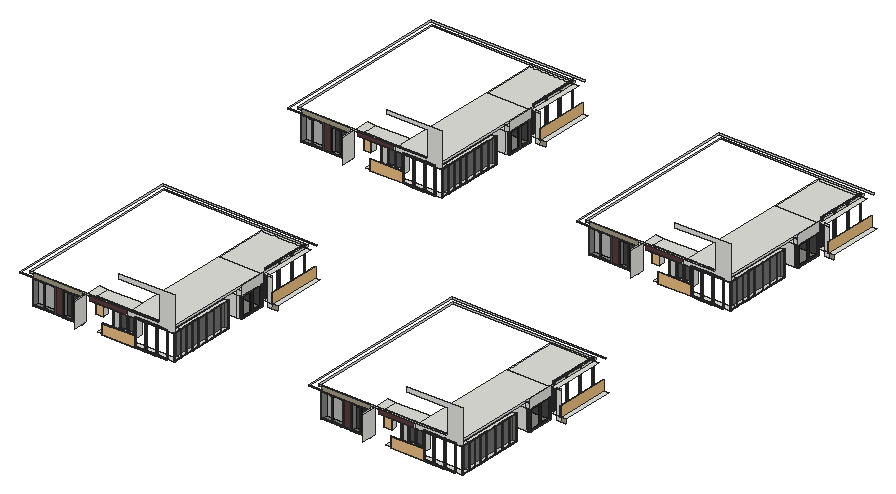
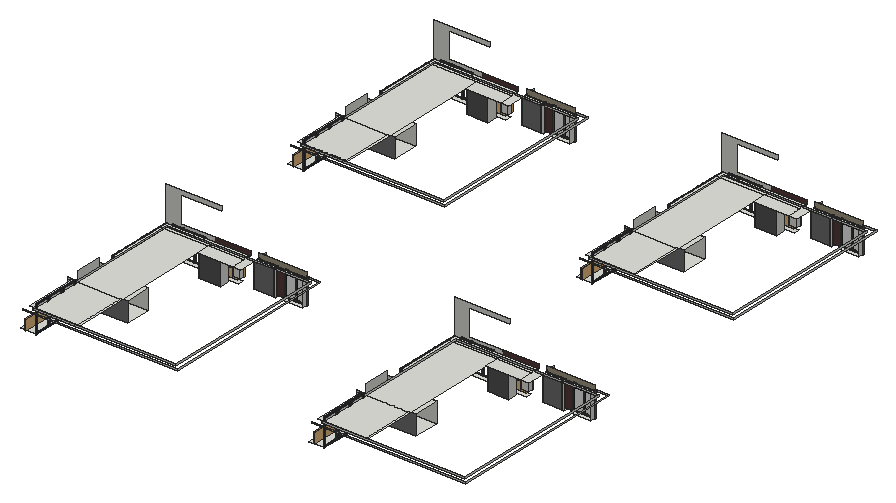
# SketchUp Ruby script. Lengths in inches.
U = 1.inch
M = Sketchup.active_model
def pt(a) = Geom::Point3d.new(a.map { |v| v * U })
def face(e, loops, mat)
  f = e.add_face(loops[0].map { |a| pt(a) })
  loops[1..].each { |l| e.add_face(l.map { |a| pt(a) }).erase! }
  f.material = f.back_material = mat if mat
  f
end
# faces: each face lists its corners as indices into pts; further lists are holes
def faces(e, pts, list, mat = nil) = list.each { |f| face(e, (f[0].is_a?(Array) ? f : [f]).map { |l| l.map { |i| pts[i] } }, mat) }
# xy, xz, yz: faces in a plane at the given z, y or x. An outline is a flat list of corners, or four numbers for a rectangle; further outlines are holes
def ring(l) = l.size == 4 ? [[l[0], l[1]], [l[2], l[1]], [l[2], l[3]], [l[0], l[3]]] : l.each_slice(2).to_a
def flat(e, list, mat, &to3) = list.each { |f| face(e, (f[0].is_a?(Array) ? f : [f]).map { |l| ring(l).map { |u, v| to3.(u, v) } }, mat) }
def xy(e, z, list, mat = nil) = flat(e, list, mat) { |x, y| [x, y, z] }
def xz(e, y, list, mat = nil) = flat(e, list, mat) { |x, z| [x, y, z] }
def yz(e, x, list, mat = nil) = flat(e, list, mat) { |y, z| [x, y, z] }
def lines(e, pts, list) = list.each { |a, b| e.add_line(pt(pts[a]), pt(pts[b])) }
# prism: a flat outline (further loops are holes) pulled along v
def prism(e, loops, v, mat = nil)
  f = face(e, loops, mat); d = Geom::Vector3d.new(v.map { |x| x * U })
  f.pushpull(f.normal.samedirection?(d) ? d.length : -d.length)
end
def box(e, o, s, mat = nil) = prism(e, [[o, [o[0] + s[0], o[1], o[2]], [o[0] + s[0], o[1] + s[1], o[2]], [o[0], o[1] + s[1], o[2]]]], [0, 0, s[2]], mat)
def at(x, y, z, deg = 0) = Geom::Transformation.translation(pt([x, y, z])) * Geom::Transformation.rotation(ORIGIN, Z_AXIS, deg.degrees)
def axes(o, x, y, z) = Geom::Transformation.new([*x, 0, *y, 0, *z, 0, *pt(o).to_a, 1])
def part(name) = M.definitions.add(name)
# library, detail: a bought-in or finely detailed component or shape, given as its bounding box
def library(name, o, s) = part(name).tap { |d| box(d.entities, o, s) }
def detail(e, o, s) = box(e.add_group.entities, o, s)
def put(e, d, t, mat = nil) = e.add_instance(d, t).tap { |i| i.material = mat if mat }
def group(e, t, mat = nil) = e.add_group.tap { |g| g.transformation = t; g.material = mat if mat }.entities
root = M.entities
M.materials.add("Glass_Tinted_Gray").color = [0, 0, 0]
M.materials["Glass_Tinted_Gray"].alpha = 0.125
M.materials.add("Glazing").color = [128, 128, 128]
M.materials["Glazing"].alpha = 0.05
M.materials.add("Powdercoating").color = [41, 44, 40]
M.materials.add("Wine2").color = [0, 0, 0]
M.materials["Wine2"].alpha = 0
M.materials.add("[0130_Gainsboro]").color = [39, 45, 50]
M.materials.add("[0135_DarkGray]").color = [81, 81, 81]
M.materials.add("[Color M05]").color = [114, 114, 114]
M.materials.add("[Color M06]").color = [86, 86, 86]
M.materials.add("[Concrete Tile]").color = [165, 155, 133]
M.materials.add("[Granite Brown]").color = [89, 59, 61]
M.materials.add("[Mirror 02]").color = [229, 229, 229]
M.materials.add("[Terrazzo Light Blue]").color = [196, 214, 227]
c1 = part("Framed glazing panel")
xy(c1.entities,0,[[0,-0.98,43.07,0],[0,0,43.07,1.4]],"[0130_Gainsboro]")
xy(c1.entities,0.3,[[0.3,-1.43,42.77,-0.98]],"[0130_Gainsboro]")
xy(c1.entities,2.95,[[2.95,-1.43,40.12,-0.63],[2.95,-0.63,40.12,0],[2.95,0,40.12,0.64],[2.95,0.64,40.12,1.4]],"[0130_Gainsboro]")
xy(c1.entities,3.54,[[3.54,-0.63,39.53,0],[3.54,0,39.53,0.64]],"[0130_Gainsboro]")
xy(c1.entities,111.8125,[[3.54,-0.63,39.53,0],[3.54,0,39.53,0.64]],"[0130_Gainsboro]")
xy(c1.entities,112.4,[[2.95,-1.43,40.12,-0.63],[2.95,-0.63,40.12,0],[2.95,0,40.12,0.64],[2.95,0.64,40.12,1.4]],"[0130_Gainsboro]")
xy(c1.entities,115.05,[[0.3,-1.43,42.77,-0.98]],"[0130_Gainsboro]")
xy(c1.entities,115.35,[[0,-0.98,43.07,0],[0,0,43.07,1.4]],"[0130_Gainsboro]")
xz(c1.entities,-1.43,[[[0.3,0.3,42.77,115.05],[2.95,2.95,40.12,112.4]]],"[0130_Gainsboro]")
xz(c1.entities,-0.98,[[[0,0,43.07,115.35],[0.3,0.3,42.77,115.05]]],"[0130_Gainsboro]")
xz(c1.entities,-0.63,[[[2.95,2.95,40.12,112.4],[3.54,3.54,39.53,111.8125]]],"[0130_Gainsboro]")
xz(c1.entities,0,[[3.54,3.54,39.53,111.8125]],"Wine2")
xz(c1.entities,0,[[[0,0,43.07,115.35],[2.95,2.95,40.12,112.4]],[[2.95,2.95,40.12,112.4],[3.54,3.54,39.53,111.8125]]],"[0130_Gainsboro]")
xz(c1.entities,0.64,[[[2.95,2.95,40.12,112.4],[3.54,3.54,39.53,111.8125]]],"[0130_Gainsboro]")
xz(c1.entities,1.4,[[[0,0,43.07,115.35],[2.95,2.95,40.12,112.4]]],"[0130_Gainsboro]")
yz(c1.entities,0,[[-0.98,0,0,115.35],[0,0,1.4,115.35]],"[0130_Gainsboro]")
yz(c1.entities,0.3,[[-1.43,0.3,-0.98,115.05]],"[0130_Gainsboro]")
yz(c1.entities,2.95,[[-1.43,2.95,-0.63,112.4],[-0.63,2.95,0,112.4],[0,2.95,0.64,112.4],[0.64,2.95,1.4,112.4]],"[0130_Gainsboro]")
yz(c1.entities,3.54,[[-0.63,3.54,0,111.8125],[0,3.54,0.64,111.8125]],"[0130_Gainsboro]")
yz(c1.entities,39.53,[[-0.63,3.54,0,111.8125],[0,3.54,0.64,111.8125]],"[0130_Gainsboro]")
yz(c1.entities,40.12,[[-1.43,2.95,-0.63,112.4],[-0.63,2.95,0,112.4],[0,2.95,0.64,112.4],[0.64,2.95,1.4,112.4]],"[0130_Gainsboro]")
yz(c1.entities,42.77,[[-1.43,0.3,-0.98,115.05]],"[0130_Gainsboro]")
yz(c1.entities,43.07,[[-0.98,0,0,115.35],[0,0,1.4,115.35]],"[0130_Gainsboro]")
c2 = part("Glazed panel assembly")
put(c2.entities,c1,axes([90.57,1.43,0],[1.05148,0,0],[0,1,0],[0,0,1]))
put(c2.entities,c1,axes([0,1.43,0],[1.05148,0,0],[0,1,0],[0,0,1]))
put(c2.entities,c1,axes([45.29,1.43,0],[1.05148,0,0],[0,1,0],[0,0,1]))
c3 = library("Glass Railing",[0,0,0],[139.5,4.76,42])
c4 = part("Group\#15")
xy(c4.entities,0,[[0,-55.94,0.71,45.94]])
xy(c4.entities,0.2,[[0,-55.94,0.47,45.94],[0.47,45.94,0.71,46.42]])
xy(c4.entities,2.36,[[0.47,-55.94,0.71,46.42]])
xz(c4.entities,-55.94,[[0,0,0.71,0,0.71,2.36,0.47,2.36,0.47,0.2,0,0.2]])
xz(c4.entities,45.94,[[0,0,0.71,0.2]])
xz(c4.entities,46.42,[[0.47,0.2,0.71,2.36]])
yz(c4.entities,0,[[-55.94,0,45.94,0.2]])
yz(c4.entities,0.47,[[-55.94,0.2,46.42,2.36]])
yz(c4.entities,0.71,[[-55.94,0,45.94,0,45.94,0.2,46.42,0.2,46.42,2.36,-55.94,2.36]])
c5 = part("Group\#7")
xy(c5.entities,0,[[0,-59.09,0.71,45.94]])
xy(c5.entities,0.2,[[0,-59.09,0.47,45.94],[0.47,45.94,0.71,46.42]])
xy(c5.entities,2.36,[[0.47,-59.09,0.71,46.42]])
xz(c5.entities,-59.09,[[0,0,0.71,0,0.71,2.36,0.47,2.36,0.47,0.2,0,0.2]])
xz(c5.entities,45.94,[[0,0,0.71,0.2]])
xz(c5.entities,46.42,[[0.47,0.2,0.71,2.36]])
yz(c5.entities,0,[[-59.09,0,45.94,0.2]])
yz(c5.entities,0.47,[[-59.09,0.2,46.42,2.36]])
yz(c5.entities,0.71,[[-59.09,0,45.94,0,45.94,0.2,46.42,0.2,46.42,2.36,-59.09,2.36]])
c6 = part("Group\#16")
prism(c6.entities,[[[0.47,-56.18,0.2],[0,-56.18,0.2],[0,-56.18,0],[0.71,-56.18,0],[0.71,-56.18,2.36],[0.47,-56.18,2.36]]],[0,28.68,0])
c7 = part("Group\#10")
box(c7.entities,[-0.73,0,0],[27.99,0.55,102.05])
c8 = part("Group\#18")
xy(c8.entities,0,[[0.47,-56.18,0.47,-55.47,0,-55.47,0,-28.21,1.18,-28.21,1.18,-56.18]])
xy(c8.entities,0.2,[[0.71,-56.18,1.18,-28.21],[0,-55.47,0.47,-28.21],[0.47,-28.21,0.71,-27.74]])
xy(c8.entities,2.36,[[0.47,-56.18,0.71,-27.74]])
xz(c8.entities,-56.18,[[0.47,0,1.18,0,1.18,0.2,0.71,0.2,0.71,2.36,0.47,2.36]])
xz(c8.entities,-55.47,[[0,0,0.47,0.2]])
xz(c8.entities,-28.21,[[0,0,1.18,0.2]])
xz(c8.entities,-27.74,[[0.47,0.2,0.71,2.36]])
yz(c8.entities,0,[[-55.47,0,-28.21,0.2]])
yz(c8.entities,0.47,[[-56.18,0,-55.47,0.2],[-56.18,0.2,-27.74,2.36]])
yz(c8.entities,0.71,[[-56.18,0.2,-27.74,2.36]])
yz(c8.entities,1.18,[[-56.18,0,-28.21,0.2]])
c9 = part("Group\#34")
xy(c9.entities,0,[[-20.45,0,7.76,1.22]])
xy(c9.entities,0.06,[[-20.39,0.06,7.7,1.22]])
xy(c9.entities,0.47,[[-19.98,0,7.28,0.06]])
xy(c9.entities,101.89,[[-19.98,0,7.28,0.06]])
xy(c9.entities,102.3,[[-20.39,0.06,7.7,1.22]])
xy(c9.entities,102.36,[[-20.45,0,7.76,1.22]])
xz(c9.entities,0,[[[-20.45,0,7.76,102.36],[-19.98,0.47,7.28,101.89]]])
xz(c9.entities,0.06,[[[-20.39,0.06,7.7,102.3],[-19.98,0.47,7.28,101.89]]])
xz(c9.entities,1.22,[[[-20.45,0,7.76,102.36],[-20.39,0.06,7.7,102.3]]])
yz(c9.entities,-20.45,[[0,0,1.22,102.36]])
yz(c9.entities,-20.39,[[0.06,0.06,1.22,102.3]])
yz(c9.entities,-19.98,[[0,0.47,0.06,101.89]])
yz(c9.entities,7.28,[[0,0.47,0.06,101.89]])
yz(c9.entities,7.7,[[0.06,0.06,1.22,102.3]])
yz(c9.entities,7.76,[[0,0,1.22,102.36]])
c10 = part("Group\#6")
put(c10.entities,c4,axes([27.97,0,7.875],[1,0,0],[0,0,-1],[0,1,0]),"Powdercoating")
put(c10.entities,c5,axes([0.71,0,6.8],[-1,0,0],[0,0,-0.97687],[0,1,0]),"Powdercoating")
put(c10.entities,c6,axes([-27.5,0,-38.07],[0,0,-1],[-1,0,0],[0,1,0]),"Powdercoating")
put(c10.entities,c7,at(1.12,0.35,-38.39),"Glazing")
put(c10.entities,c8,axes([-27.5,0,63.35],[0,0,1],[-1,0,0],[0,1,0]),"Powdercoating")
put(c10.entities,c9,at(20.6875,1.0625,-38.54),"Powdercoating")
c11 = part("Sliding door assembly")
put(c11.entities,c10,at(-1.18,4.5,38.86))
g1 = group(c11.entities,at(84.74,4.5,38.86))
put(g1,c4,axes([-27.97,0,7.875],[-1,0,0],[0,0,-1],[0,1,0]),"Powdercoating")
put(g1,c5,axes([-0.71,0,6.8],[1,0,0],[0,0,-0.97687],[0,1,0]),"Powdercoating")
put(g1,c6,axes([27.5,0,-38.07],[0,0,-1],[1,0,0],[0,1,0]),"Powdercoating")
put(g1,c7,axes([-1.12,0.35,-38.39],[-1,0,0],[0,1,0],[0,0,1]),"Glazing")
put(g1,c8,axes([27.5,0,63.35],[0,0,1],[1,0,0],[0,1,0]),"Powdercoating")
put(g1,c9,axes([-20.6875,1.0625,-38.54],[-1,0,0],[0,1,0],[0,0,1]),"Powdercoating")
g2 = group(c11.entities,at(56.0625,4.5,38.86))
put(g2,c4,axes([-27.97,0,7.875],[-1,0,0],[0,0,-1],[0,1,0]),"Powdercoating")
put(g2,c6,axes([27.5,0,-38.07],[0,0,-1],[1,0,0],[0,1,0]),"Powdercoating")
put(g2,c7,axes([-1.12,0.35,-38.39],[-1,0,0],[0,1,0],[0,0,1]),"Glazing")
put(g2,c8,axes([27.5,0,63.35],[0,0,1],[1,0,0],[0,1,0]),"Powdercoating")
put(g2,c9,axes([-20.6875,1.0625,-38.54],[-1,0,0],[0,1,0],[0,0,1]),"Powdercoating")
g3 = group(g2,at(-0.71,0,6.8),"Powdercoating")
xy(g3,-45.34,[[0.47,0.2,0.71,2.36]])
xy(g3,-44.88,[[0,0,0.71,0.2]])
xy(g3,57.73,[[0,0,0.71,0,0.71,2.36,0.47,2.36,0.47,0.2,0,0.2]])
xz(g3,0,[[0,-44.88,0.71,57.73]])
xz(g3,0.2,[[0.47,-45.34,0.71,-44.88],[0,-44.88,0.47,57.73]])
xz(g3,2.36,[[0.47,-45.34,0.71,57.73]])
yz(g3,0,[[0,-44.88,0.2,57.73]])
yz(g3,0.47,[[0.2,-45.34,2.36,57.73]])
yz(g3,0.71,[[0.2,-45.34,2.36,-45.34,2.36,57.73,0,57.73,0,-44.88,0.2,-44.88]])
put(c11.entities,c10,axes([-33.94,4.5,38.86],[1.14218,0,0],[0,1,0],[0,0,1]))
c12 = part("sliding door")
put(c12.entities,c11,at(0,-4.5,-0.08))
c13 = part("PENTEK_RP Fineline 50S_Sliding_DoorCase_E1")
box(c13.entities,[0,0,0],[1.51,3.66,99.27],"[0135_DarkGray]")
c14 = part("PENTEK_RP Fineline 50S_SlidingDooe_Case_E2")
box(c14.entities,[0,0,0],[96.25,3.66,1.51],"[0135_DarkGray]")
c15 = part("pentek_RP Fineline 50S_SlidingDoor_Case")
put(c15.entities,c13,at(97.76,0,0))
put(c15.entities,c14,at(1.51,0,0))
put(c15.entities,c13,at(0,0,0))
put(c15.entities,c14,at(1.51,0,97.76))
c16 = part("PENTEK_RP Fineline 50S_SlidingDoor_GlazingBead_2")
box(c16.entities,[0,0,0],[0.56,0.59,94.39],"[0135_DarkGray]")
c17 = part("PENTEK_RP Fineline 50S_SlidingDoor_Glass")
box(c17.entities,[0,0,0],[46.58,0.16,94.39],"Glass_Tinted_Gray")
c18 = part("PENTEK_RP Fineline 50S_SlidingDoor_GlazingBead")
box(c18.entities,[0,0,0],[45.47,0.59,0.56],"[0135_DarkGray]")
c19 = part("PENTEK_RP Fineline 50S_SlidingDoor_Leaf_E1")
xy(c19.entities,0,[[0,0,0.93,1.97],[0.93,1.57,1.49,1.97]],"[0135_DarkGray]")
xy(c19.entities,96.25,[[0,0,0.93,0,0.93,1.57,1.49,1.57,1.49,1.97,0,1.97]],"[0135_DarkGray]")
xz(c19.entities,0,[[0,0,0.93,96.25]],"[0135_DarkGray]")
xz(c19.entities,1.57,[[0.93,0,1.49,95.32],[0.93,95.32,1.49,96.25]],"[0135_DarkGray]")
xz(c19.entities,1.97,[[0,0,1.49,96.25]],"[0135_DarkGray]")
yz(c19.entities,0,[[0,0,1.97,96.25]],"[0135_DarkGray]")
yz(c19.entities,0.93,[[0,0,1.57,0.93],[0,0.93,1.57,95.32],[0,95.32,1.57,96.25]],"[0135_DarkGray]")
yz(c19.entities,1.49,[[1.57,0,1.97,95.32],[1.57,95.32,1.97,96.25]],"[0135_DarkGray]")
c20 = part("PENTEK_RP Fineline 50S_SlidingDoor_Leaf_E2")
xy(c20.entities,0,[[0,0,0,1.57,0.56,1.57,0.56,1.97,46.02,1.97,46.02,1.57,46.58,1.57,46.58,0]],"[0135_DarkGray]")
xy(c20.entities,0.93,[[0,0,46.58,1.57]],"[0135_DarkGray]")
xy(c20.entities,1.49,[[0.56,1.57,46.02,1.97]],"[0135_DarkGray]")
xz(c20.entities,0,[[0,0,46.58,0.93]],"[0135_DarkGray]")
xz(c20.entities,1.57,[[0,0,0.56,0.93],[46.02,0,46.58,0.93],[0.56,0.93,46.02,1.49]],"[0135_DarkGray]")
xz(c20.entities,1.97,[[0.56,0,46.02,1.49]],"[0135_DarkGray]")
yz(c20.entities,0,[[0,0,1.57,0.93]],"[0135_DarkGray]")
yz(c20.entities,0.56,[[1.57,0,1.97,0.93],[1.57,0.93,1.97,1.49]],"[0135_DarkGray]")
yz(c20.entities,46.02,[[1.57,0,1.97,0.93],[1.57,0.93,1.97,1.49]],"[0135_DarkGray]")
yz(c20.entities,46.58,[[0,0,1.57,0.93]],"[0135_DarkGray]")
c21 = part("PENTEK_RP Fineline S_SlidingDoor_Leaf1")
put(c21.entities,c16,at(0.93,0,0.93))
put(c21.entities,c16,at(46.96,0,0.93))
put(c21.entities,c17,at(1.49,1.42,0.93))
put(c21.entities,c18,at(1.49,0,0.93))
put(c21.entities,c17,at(1.49,0.59,0.93),"[Terrazzo Light Blue]")
put(c21.entities,c19,at(0,0,0))
put(c21.entities,c19,axes([48.44,0,0],[-1,0,0],[0,1,0],[0,0,1]))
put(c21.entities,c20,axes([0.93,0,96.25],[1,0,0],[0,1,0],[0,0,-1]))
put(c21.entities,c20,at(0.93,0,0))
put(c21.entities,c18,at(1.49,0,94.77))
c22 = part("PENTEK_RP Fineline 50S_SlidingDoor_Leaf2")
put(c22.entities,c17,at(1.49,1.42,0.93))
put(c22.entities,c18,at(1.49,0,94.77))
put(c22.entities,c16,at(46.96,0,0.93))
put(c22.entities,c17,at(1.49,0.59,0.93),"[Mirror 02]")
put(c22.entities,c16,at(0.93,0,0.93))
put(c22.entities,c19,at(0,0,0))
put(c22.entities,c19,axes([48.44,0,0],[-1,0,0],[0,1,0],[0,0,1]))
put(c22.entities,c18,at(1.49,0,0.93))
put(c22.entities,c20,axes([0.93,0,96.25],[1,0,0],[0,1,0],[0,0,-1]))
put(c22.entities,c20,at(0.93,0,0))
c23 = part("PENTEK - Slimmest Steel Sliding Door / Window\#1")
put(c23.entities,c15,at(0,-1.88,-0.09))
put(c23.entities,c21,at(1.51,-2.27,1.42))
put(c23.entities,c22,at(49.32,-0.3,1.42))
c24 = library("Klein+raam",[128.36,12.7,0],[19.68,5.51,55.12])
xy(root,1276.95,[[646.53,1835.1875,662.84,1873.375],[662.84,1835.1875,664.52,1873.375],[664.52,1835.1875,715.63,1873.375],[1864.72,1835.1875,1881.02,1873.375],[1881.02,1835.1875,1882.71,1873.375],
  [1882.71,1835.1875,1933.82,1873.375],[646.53,3249.875,662.84,3288.0625],[662.84,3249.875,664.52,3288.0625],[664.52,3249.875,715.63,3288.0625],[1864.72,3249.875,1881.02,3288.0625],
  [1881.02,3249.875,1882.71,3288.0625],[1882.71,3249.875,1933.82,3288.0625]])
xy(root,1277.26,[[625.7,1835.1875,646.53,1873.375],[1843.88,1835.1875,1864.72,1873.375],[625.7,3249.875,646.53,3288.0625],[1843.88,3249.875,1864.72,3288.0625]])
xy(root,1278.6875,[[589.79,1799.9375,913.875,1799.9375,913.875,1835.1875,890.875,1835.1875,890.875,1822.9375,589.79,1822.9375],[1807.98,1799.9375,2132.0625,1799.9375,2132.0625,1835.1875,2109.0625,1835.1875,2109.0625,1822.9375,1807.98,1822.9375],[894.3125,1835.1875,913.875,2085.72],[2112.5,1835.1875,2132.0625,2085.72],[589.79,3214.625,913.875,3214.625,913.875,3249.875,890.875,3249.875,890.875,3237.625,589.79,3237.625],
  [1807.98,3214.625,2132.0625,3214.625,2132.0625,3249.875,2109.0625,3249.875,2109.0625,3237.625,1807.98,3237.625],[894.3125,3249.875,913.875,3500.41],[2112.5,3249.875,2132.0625,3500.41]])
xy(root,1281.4375,[[319.53,1799.9375,523.04,1799.9375,523.04,1822.9375,442.15,1822.9375,442.15,1806.5625,404.95,1806.5625,404.95,1822.9375,319.53,1822.9375],[1537.72,1799.9375,1741.23,1799.9375,1741.23,1822.9375,1660.33,1822.9375,1660.33,1806.5625,1623.14,1806.5625,1623.14,1822.9375,1537.72,1822.9375],[431.33,1806.5625,442.15,1822.9375],[1649.52,1806.5625,1660.33,1822.9375],[319.53,3214.625,523.04,3214.625,523.04,3237.625,442.15,3237.625,442.15,3221.25,404.95,3221.25,404.95,3237.625,319.53,3237.625],
  [1537.72,3214.625,1741.23,3214.625,1741.23,3237.625,1660.33,3237.625,1660.33,3221.25,1623.14,3221.25,1623.14,3237.625,1537.72,3237.625],[431.33,3221.25,442.15,3237.625],[1649.52,3221.25,1660.33,3237.625]])
xy(root,1283.36,[[704.25,2156.01,913.875,2266.33],[1922.4375,2156.01,2132.0625,2266.33],[704.25,3570.7,913.875,3681.01],[1922.4375,3570.7,2132.0625,3681.01]])
xy(root,1286.8125,[[890.875,2295.875,954.6875,2518.89],[2109.0625,2295.875,2172.875,2518.89],[890.875,3710.5625,954.6875,3933.57],[2109.0625,3710.5625,2172.875,3933.57]])
xy(root,1321.04,[[557.4,1835.1875,588.66,1854.3125],[1775.59,1835.1875,1806.84,1854.3125],[557.4,3249.875,588.66,3269],[1775.59,3249.875,1806.84,3269]])
xy(root,1369.04,[[704.25,2156.01,913.875,2266.33],[1922.4375,2156.01,2132.0625,2266.33],[704.25,3570.7,913.875,3681.01],[1922.4375,3570.7,2132.0625,3681.01]])
xy(root,1373.32,[[557.4,1835.1875,588.66,1854.3125],[1775.59,1835.1875,1806.84,1854.3125],[557.4,3249.875,588.66,3269],[1775.59,3249.875,1806.84,3269]])
xy(root,1375.08,[[625.7,1835.1875,715.63,1873.375],[1843.88,1835.1875,1933.82,1873.375],[625.7,3249.875,715.63,3288.0625],[1843.88,3249.875,1933.82,3288.0625]])
xy(root,1386,[[319.53,1799.9375,319.53,1822.9375,405.55,1822.9375,405.55,1806.5625,442.15,1806.5625,442.15,1822.9375,523.04,1822.9375,523.04,1799.9375],[557.88,1799.9375,557.88,1822.9375,890.875,1822.9375,890.875,1835.1875,913.875,1835.1875,913.875,1799.9375],[1537.72,1799.9375,1537.72,1822.9375,1623.74,1822.9375,1623.74,1806.5625,1660.33,1806.5625,1660.33,1822.9375,1741.23,1822.9375,1741.23,1799.9375],[1776.07,1799.9375,1776.07,1822.9375,2109.0625,1822.9375,2109.0625,1835.1875,2132.0625,1835.1875,2132.0625,1799.9375],[431.33,1806.5625,442.15,1822.9375],
  [1649.52,1806.5625,1660.33,1822.9375],[523.04,1822.9375,557.88,1822.9375,557.88,1835.1875,557.4,1835.1875,557.4,1893.6875,523.04,1893.6875],[557.88,1822.9375,704.25,1835.1875],[704.25,1822.9375,890.875,1835.1875],[1741.23,1822.9375,1776.07,1822.9375,1776.07,1835.1875,1775.59,1835.1875,1775.59,1893.6875,1741.23,1893.6875],
  [1776.07,1822.9375,1922.4375,1835.1875],[1922.4375,1822.9375,2109.0625,1835.1875],[557.4,1835.1875,704.25,1893.6875],[704.25,1835.1875,890.875,2295.875],[894.3125,1835.1875,913.875,2085.72],
  [1775.59,1835.1875,1922.4375,1893.6875],[1922.4375,1835.1875,2109.0625,2295.875],[2112.5,1835.1875,2132.0625,2085.72],[704.25,2295.875,710.125,2518.89],[710.125,2295.875,890.875,2518.89],
  [890.875,2295.875,913.875,2518.89],[1922.4375,2295.875,1928.3125,2518.89],[1928.3125,2295.875,2109.0625,2518.89],[2109.0625,2295.875,2132.0625,2518.89],[704.25,2518.89,890.875,2531.375],
  [1922.4375,2518.89,2109.0625,2531.375],[319.53,3214.625,319.53,3237.625,405.55,3237.625,405.55,3221.25,442.15,3221.25,442.15,3237.625,523.04,3237.625,523.04,3214.625],[557.88,3214.625,557.88,3237.625,890.875,3237.625,890.875,3249.875,913.875,3249.875,913.875,3214.625],[1537.72,3214.625,1537.72,3237.625,1623.74,3237.625,1623.74,3221.25,1660.33,3221.25,1660.33,3237.625,1741.23,3237.625,1741.23,3214.625],[1776.07,3214.625,1776.07,3237.625,2109.0625,3237.625,2109.0625,3249.875,2132.0625,3249.875,2132.0625,3214.625],
  [431.33,3221.25,442.15,3237.625],[1649.52,3221.25,1660.33,3237.625],[523.04,3237.625,557.88,3237.625,557.88,3249.875,557.4,3249.875,557.4,3308.375,523.04,3308.375],[557.88,3237.625,704.25,3249.875],[704.25,3237.625,890.875,3249.875],
  [1741.23,3237.625,1776.07,3237.625,1776.07,3249.875,1775.59,3249.875,1775.59,3308.375,1741.23,3308.375],[1776.07,3237.625,1922.4375,3249.875],[1922.4375,3237.625,2109.0625,3249.875],[557.4,3249.875,704.25,3308.375],[704.25,3249.875,890.875,3710.5625],
  [894.3125,3249.875,913.875,3500.41],[1775.59,3249.875,1922.4375,3308.375],[1922.4375,3249.875,2109.0625,3710.5625],[2112.5,3249.875,2132.0625,3500.41],[704.25,3710.5625,710.125,3933.57],
  [710.125,3710.5625,890.875,3933.57],[890.875,3710.5625,913.875,3933.57],[1922.4375,3710.5625,1928.3125,3933.57],[1928.3125,3710.5625,2109.0625,3933.57],[2109.0625,3710.5625,2132.0625,3933.57],
  [704.25,3933.57,890.875,3946.0625],[1922.4375,3933.57,2109.0625,3946.0625]])
xz(root,1799.9375,[[262.875,1386,319.53,1392],[708.87,1386,913.875,1386,913.875,1530.6875,679.51,1530.6875,679.51,1512,851.78,1512,851.78,1404.6875,708.87,1404.6875],[1481.0625,1386,1537.72,1392],[1927.06,1386,2132.0625,1386,2132.0625,1530.6875,1897.7,1530.6875,1897.7,1512,2069.97,1512,2069.97,1404.6875,1927.06,1404.6875]])
xz(root,1799.9375,[[319.53,1386,523.04,1407.4375],[1537.72,1386,1741.23,1407.4375]],"[Concrete Tile]")
xz(root,1799.9375,[[557.88,1386,708.87,1404.6875],[1776.07,1386,1927.06,1404.6875]],"[Granite Brown]")
xz(root,1806.5625,[[405.03,1281.4375,442.15,1281.4375,442.15,1386,405.55,1386],[1623.22,1281.4375,1660.33,1281.4375,1660.33,1386,1623.74,1386]],"[Granite Brown]")
xz(root,1822.9375,[[431.33,1281.4375,442.15,1386],[1649.52,1281.4375,1660.33,1386],[285.875,1386,890.875,1392],[1504.0625,1386,2109.0625,1392]])
xz(root,1822.9375,[[442.15,1281.4375,523.04,1386],[1660.33,1281.4375,1741.23,1386]],"[Color M05]")
xz(root,1835.1875,[[556.34,1321.04,557.4,1373.32],[1774.53,1321.04,1775.59,1373.32]])
xz(root,1835.1875,[[557.4,1321.04,557.88,1373.32],[1775.59,1321.04,1776.07,1373.32]],"[Granite Brown]")
xz(root,1854.3125,[[557.4,1321.04,588.66,1373.32],[1775.59,1321.04,1806.84,1373.32]])
xz(root,1873.375,[[646.53,1276.95,715.63,1276.95,715.63,1375.08,625.7,1375.08,625.7,1277.26,646.53,1277.26],[1864.72,1276.95,1933.82,1276.95,1933.82,1375.08,1843.88,1375.08,1843.88,1277.26,1864.72,1277.26]],"[Color M06]")
xz(root,2085.72,[[894.3125,1278.6875,913.875,1386],[2112.5,1278.6875,2132.0625,1386]],"[Color M05]")
xz(root,2156.01,[[704.25,1283.36,894.3125,1369.04],[894.3125,1283.36,913.875,1369.04],[1922.4375,1283.36,2112.5,1369.04],[2112.5,1283.36,2132.0625,1369.04],[2112.5,1283.36,2132.0625,1369.04],
  [894.3125,1369.04,913.875,1392],[2112.5,1369.04,2132.0625,1392]])
xz(root,2266.33,[[704.25,1283.36,913.875,1369.04],[1922.4375,1283.36,2132.0625,1369.04]],"[Color M05]")
xz(root,2295.875,[[913.875,1267.75,930.75,1286.8125],[2132.0625,1267.75,2148.9375,1286.8125],[913.875,1286.8125,930.75,1386],[2132.0625,1286.8125,2148.9375,1386],[913.875,1386,930.75,1392],
  [2132.0625,1386,2148.9375,1392]])
xz(root,2295.875,[[930.75,1267.75,954.6875,1286.8125],[2148.9375,1267.75,2172.875,1286.8125]],"[Concrete Tile]")
xz(root,2531.375,[[285.875,1386,890.875,1392],[1504.0625,1386,2109.0625,1392]])
xz(root,2554.375,[[262.875,1386,913.875,1392],[1481.0625,1386,2132.0625,1392]])
xz(root,3214.625,[[262.875,1386,319.53,1392],[708.87,1386,913.875,1386,913.875,1530.6875,679.51,1530.6875,679.51,1512,851.78,1512,851.78,1404.6875,708.87,1404.6875],[1481.0625,1386,1537.72,1392],[1927.06,1386,2132.0625,1386,2132.0625,1530.6875,1897.7,1530.6875,1897.7,1512,2069.97,1512,2069.97,1404.6875,1927.06,1404.6875]])
xz(root,3214.625,[[319.53,1386,523.04,1407.4375],[1537.72,1386,1741.23,1407.4375]],"[Concrete Tile]")
xz(root,3214.625,[[557.88,1386,708.87,1404.6875],[1776.07,1386,1927.06,1404.6875]],"[Granite Brown]")
xz(root,3221.25,[[405.03,1281.4375,442.15,1281.4375,442.15,1386,405.55,1386],[1623.22,1281.4375,1660.33,1281.4375,1660.33,1386,1623.74,1386]],"[Granite Brown]")
xz(root,3237.625,[[431.33,1281.4375,442.15,1386],[1649.52,1281.4375,1660.33,1386],[285.875,1386,890.875,1392],[1504.0625,1386,2109.0625,1392]])
xz(root,3237.625,[[442.15,1281.4375,523.04,1386],[1660.33,1281.4375,1741.23,1386]],"[Color M05]")
xz(root,3249.875,[[556.34,1321.04,557.4,1373.32],[1774.53,1321.04,1775.59,1373.32]])
xz(root,3249.875,[[557.4,1321.04,557.88,1373.32],[1775.59,1321.04,1776.07,1373.32]],"[Granite Brown]")
xz(root,3269,[[557.4,1321.04,588.66,1373.32],[1775.59,1321.04,1806.84,1373.32]])
xz(root,3288.0625,[[646.53,1276.95,715.63,1276.95,715.63,1375.08,625.7,1375.08,625.7,1277.26,646.53,1277.26],[1864.72,1276.95,1933.82,1276.95,1933.82,1375.08,1843.88,1375.08,1843.88,1277.26,1864.72,1277.26]],"[Color M06]")
xz(root,3500.41,[[894.3125,1278.6875,913.875,1386],[2112.5,1278.6875,2132.0625,1386]],"[Color M05]")
xz(root,3570.7,[[704.25,1283.36,894.3125,1369.04],[894.3125,1283.36,913.875,1369.04],[1922.4375,1283.36,2112.5,1369.04],[2112.5,1283.36,2132.0625,1369.04],[894.3125,1369.04,913.875,1392],
  [2112.5,1369.04,2132.0625,1392]])
xz(root,3681.01,[[704.25,1283.36,913.875,1369.04],[1922.4375,1283.36,2132.0625,1369.04]],"[Color M05]")
xz(root,3710.5625,[[913.875,1267.75,930.75,1286.8125],[2132.0625,1267.75,2148.9375,1286.8125],[913.875,1286.8125,930.75,1386],[2132.0625,1286.8125,2148.9375,1386],[913.875,1386,930.75,1392],
  [2132.0625,1386,2148.9375,1392]])
xz(root,3710.5625,[[930.75,1267.75,954.6875,1286.8125],[2148.9375,1267.75,2172.875,1286.8125]],"[Concrete Tile]")
xz(root,3946.0625,[[285.875,1386,890.875,1392],[1504.0625,1386,2109.0625,1392]])
xz(root,3969.0625,[[262.875,1386,913.875,1392],[1481.0625,1386,2132.0625,1392]])
yz(root,262.875,[[1799.9375,1386,2554.375,1392],[3214.625,1386,3969.0625,1392]])
yz(root,285.875,[[1822.9375,1386,2531.375,1392],[3237.625,1386,3946.0625,1392]])
yz(root,319.53,[[1799.9375,1281.4375,1822.9375,1386],[3214.625,1281.4375,3237.625,1386]])
yz(root,442.15,[[1806.5625,1281.4375,1822.9375,1386],[3221.25,1281.4375,3237.625,1386]])
yz(root,523.04,[[1763.25,1281.4375,1822.9375,1386],[3177.9375,1281.4375,3237.625,1386],[1763.25,1386,1799.9375,1392],[3177.9375,1386,3214.625,1392]])
yz(root,557.4,[[1835.1875,1321.04,1854.3125,1373.32],[3249.875,1321.04,3269,1373.32]])
yz(root,588.66,[[1835.1875,1321.04,1854.3125,1373.32],[3249.875,1321.04,3269,1373.32]])
yz(root,625.7,[[1835.1875,1277.26,1873.375,1375.08],[3249.875,1277.26,3288.0625,1375.08]])
yz(root,646.53,[[1835.1875,1276.95,1873.375,1277.26],[3249.875,1276.95,3288.0625,1277.26]])
yz(root,715.63,[[1835.1875,1276.95,1873.375,1375.08],[3249.875,1276.95,3288.0625,1375.08]])
yz(root,890.875,[[1822.9375,1386,2531.375,1392],[3237.625,1386,3946.0625,1392]])
yz(root,894.3125,[[1835.1875,1278.6875,2085.72,1386],[3249.875,1278.6875,3500.41,1386]],"[Color M05]")
yz(root,913.875,[[2156.01,1369.04,2266.33,1409.36],[3570.7,1369.04,3681.01,1409.36]])
yz(root,1481.0625,[[1799.9375,1386,2554.375,1392],[3214.625,1386,3969.0625,1392]])
yz(root,1504.0625,[[1822.9375,1386,2531.375,1392],[3237.625,1386,3946.0625,1392]])
yz(root,1537.72,[[1799.9375,1281.4375,1822.9375,1386],[3214.625,1281.4375,3237.625,1386]])
yz(root,1660.33,[[1806.5625,1281.4375,1822.9375,1386],[3221.25,1281.4375,3237.625,1386]])
yz(root,1741.23,[[1763.25,1281.4375,1822.9375,1386],[3177.9375,1281.4375,3237.625,1386],[1763.25,1386,1799.9375,1392],[3177.9375,1386,3214.625,1392]])
yz(root,1775.59,[[1835.1875,1321.04,1854.3125,1373.32],[3249.875,1321.04,3269,1373.32]])
yz(root,1806.84,[[1835.1875,1321.04,1854.3125,1373.32],[3249.875,1321.04,3269,1373.32]])
yz(root,1843.88,[[1835.1875,1277.26,1873.375,1375.08],[3249.875,1277.26,3288.0625,1375.08]])
yz(root,1864.72,[[1835.1875,1276.95,1873.375,1277.26],[3249.875,1276.95,3288.0625,1277.26]])
yz(root,1933.82,[[1835.1875,1276.95,1873.375,1375.08],[3249.875,1276.95,3288.0625,1375.08]])
yz(root,2109.0625,[[1822.9375,1386,2531.375,1392],[3237.625,1386,3946.0625,1392]])
yz(root,2112.5,[[1835.1875,1278.6875,2085.72,1386],[3249.875,1278.6875,3500.41,1386]],"[Color M05]")
yz(root,2132.0625,[[2156.01,1369.04,2266.33,1409.36],[3570.7,1369.04,3681.01,1409.36]])
p = [[1933.82,1798.76,1404.6875],[1933.82,1798.76,1386],[715.63,1798.76,1404.6875],[715.63,1798.76,1386],[1933.82,3213.45,1404.6875],[1933.82,3213.45,1386],
  [715.63,3213.45,1404.6875],[715.63,3213.45,1386]]
lines(root,p,[[0,1],[2,3],[4,5],[6,7]])
put(root,c2,at(1966.3,1799.14,1275.15))
put(root,c2,at(748.11,1799.14,1275.15))
put(root,c2,at(1966.3,3213.83,1275.15))
put(root,c2,at(748.11,3213.83,1275.15))
put(root,c3,at(1827.12,1799.14,1275.45))
put(root,c3,at(608.93,1799.14,1275.45))
put(root,c3,at(1827.12,3213.83,1275.45))
put(root,c3,at(608.93,3213.83,1275.45))
put(root,c12,axes([2132.0625,1973.09,1278.6875],[0,1.302,0],[-1,0,0],[0,0,1.03877]))
put(root,c12,axes([913.875,1973.09,1278.6875],[0,1.302,0],[-1,0,0],[0,0,1.03877]))
put(root,c12,axes([2132.0625,3387.78,1278.6875],[0,1.302,0],[-1,0,0],[0,0,1.03877]))
put(root,c12,axes([913.875,3387.78,1278.6875],[0,1.302,0],[-1,0,0],[0,0,1.03877]))
put(root,c12,axes([2132.0625,1836.17,1278.6875],[0,1.06764,0],[-1,0,0],[0,0,1.03877]))
put(root,c12,axes([913.875,1836.17,1278.6875],[0,1.06764,0],[-1,0,0],[0,0,1.03877]))
put(root,c12,axes([2132.0625,3250.86,1278.6875],[0,1.06764,0],[-1,0,0],[0,0,1.03877]))
put(root,c12,axes([913.875,3250.86,1278.6875],[0,1.06764,0],[-1,0,0],[0,0,1.03877]))
put(root,c23,axes([1659.95,1801.59,1281.53],[0.81876,0,0],[0,0.88,0],[0,0,1.054]))
put(root,c23,axes([441.76,1801.59,1281.53],[0.81876,0,0],[0,0.88,0],[0,0,1.054]))
put(root,c23,axes([1659.95,3216.28,1281.53],[0.81876,0,0],[0,0.88,0],[0,0,1.054]))
put(root,c23,axes([441.76,3216.28,1281.53],[0.81876,0,0],[0,0.88,0],[0,0,1.054]))
put(root,c23,axes([1534.57,1801.59,1281.53],[0.94111,0,0],[0,0.88,0],[0,0,1.054]))
put(root,c23,axes([316.38,1801.59,1281.53],[0.94111,0,0],[0,0.88,0],[0,0,1.054]))
put(root,c23,axes([1534.57,3216.28,1281.53],[0.94111,0,0],[0,0.88,0],[0,0,1.054]))
put(root,c23,axes([316.38,3216.28,1281.53],[0.94111,0,0],[0,0.88,0],[0,0,1.054]))
put(root,c23,axes([2127.34,2156.65,1283.4375],[0,1.12181,0],[-2.51374,0,0],[0,0,0.87918]))
put(root,c23,axes([909.16,2156.65,1283.4375],[0,1.12181,0],[-2.51374,0,0],[0,0,0.87918]))
put(root,c23,axes([2127.34,3571.34,1283.4375],[0,1.12181,0],[-2.51374,0,0],[0,0,0.87918]))
put(root,c23,axes([909.16,3571.34,1283.4375],[0,1.12181,0],[-2.51374,0,0],[0,0,0.87918]))
put(root,c2,axes([2109.0625,2310.05,1286.51],[0,1.54079,0],[-1,0,0],[0,0,1]))
put(root,c2,axes([890.875,2310.05,1286.51],[0,1.54079,0],[-1,0,0],[0,0,1]))
put(root,c2,axes([2109.0625,3724.73,1286.51],[0,1.54079,0],[-1,0,0],[0,0,1]))
put(root,c2,axes([890.875,3724.73,1286.51],[0,1.54079,0],[-1,0,0],[0,0,1]))
put(root,c3,axes([2152.47,2295.6875,1286.8125],[0,1.6,0],[-1,0,0],[0,0,1]))
put(root,c3,axes([934.28,2295.6875,1286.8125],[0,1.6,0],[-1,0,0],[0,0,1]))
put(root,c3,axes([2152.47,3710.375,1286.8125],[0,1.6,0],[-1,0,0],[0,0,1]))
put(root,c3,axes([934.28,3710.375,1286.8125],[0,1.6,0],[-1,0,0],[0,0,1]))
put(root,c2,axes([1845.55,1835.1875,1290.79],[0.6649,0,0],[0,0.61,0],[0,0,0.74986]),"[Color M06]")
put(root,c2,axes([627.36,1835.1875,1290.79],[0.6649,0,0],[0,0.61,0],[0,0,0.74986]),"[Color M06]")
put(root,c2,axes([1845.55,3249.875,1290.79],[0.6649,0,0],[0,0.61,0],[0,0,0.74986]),"[Color M06]")
put(root,c2,axes([627.36,3249.875,1290.79],[0.6649,0,0],[0,0.61,0],[0,0,0.74986]),"[Color M06]")
put(root,c24,axes([1571.78,1822.81,1321.04],[1.58777,0,0],[0,0.68,0],[0,0,0.99202]))
put(root,c24,axes([353.6,1822.81,1321.04],[1.58777,0,0],[0,0.68,0],[0,0,0.99202]))
put(root,c24,axes([1571.78,3237.49,1321.04],[1.58777,0,0],[0,0.68,0],[0,0,0.99202]))
put(root,c24,axes([353.6,3237.49,1321.04],[1.58777,0,0],[0,0.68,0],[0,0,0.99202]))
